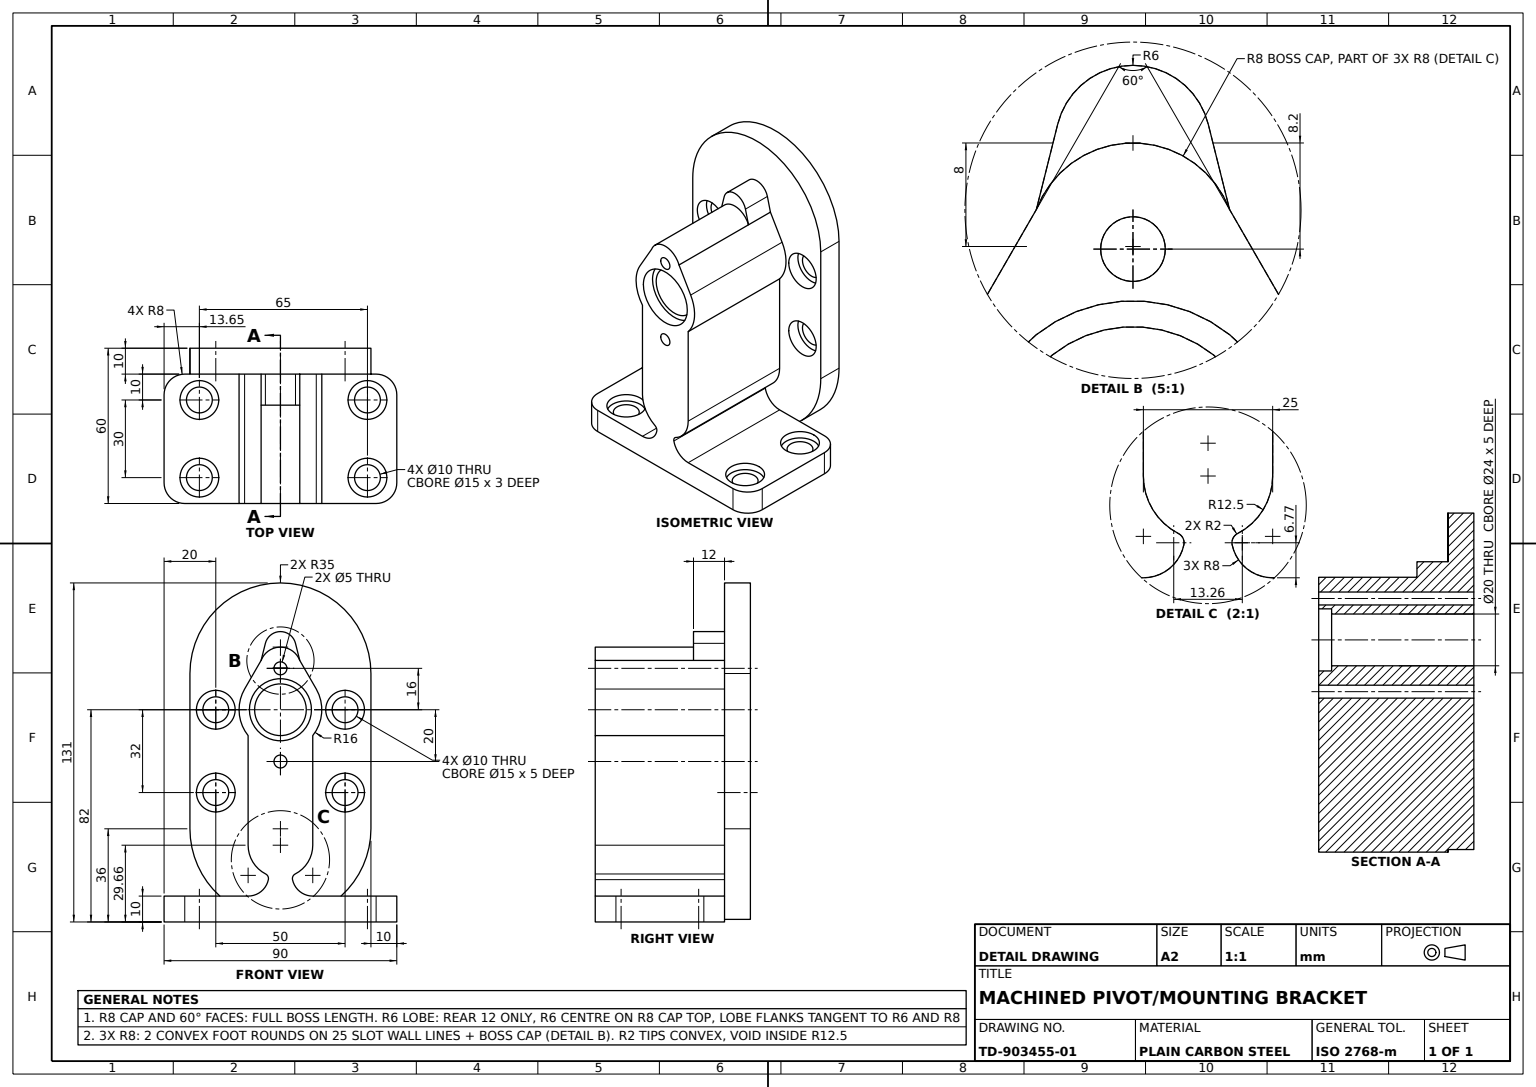
solid
v1 (-16,0,60)
v2 (-16,0,10)
e1 v1 v2 LINE
v3 (-13.856406,8,60)
e2 v3 v1 CIRCLE(AX(P(0,0,60),D(0,0,1),D(1,0,0)),16)
v4 (-13.856406,8,10)
e3 v3 v4 LINE
e4 v4 v2 CIRCLE(AX(P(0,0,10),D(0,0,1),D(1,0,0)),16)
face CYL(AX(P(0,0,60),D(0,0,-1),D(-1,0,0)),16) [-e1 -e2 e3 e4]
v5 (30,0,5)
v6 (20,0,5)
e5 v5 v6 CIRCLE(AX(P(25,0,5),D(0,0,1),D(1,0,0)),5)
e6 v6 v5 CIRCLE(AX(P(25,0,5),D(0,0,1),D(1,0,0)),5)
v7 (32.5,0,5)
v8 (17.5,0,5)
e7 v7 v8 CIRCLE(AX(P(25,0,5),D(0,0,1),D(1,0,0)),7.5)
e8 v8 v7 CIRCLE(AX(P(25,0,5),D(0,0,1),D(1,0,0)),7.5)
face PLANE(AX(P(25,0,5),D(0,0,1),D(1,0,0))) [-e5 -e6] [e7 e8]
v9 (7.473379,19.055728,22)
v10 (7.473379,19.055728,10)
e9 v9 v10 LINE
v11 (5.820364,25.658327,10)
e10 v10 v11 LINE
v12 (5.820364,25.658327,22)
e11 v12 v11 LINE
e12 v9 v12 LINE
face PLANE(AX(P(7.473379,19.055728,22),D(-0.970060689,-0.242862635,0),D(0.242862635,-0.970060689,0))) rev [e9 e10 -e11 -e12]
v13 (2.5,-20,60)
v14 (-2.5,-20,60)
e13 v13 v14 CIRCLE(AX(P(0,-20,60),D(0,0,1),D(1,0,0)),2.5)
e14 v14 v13 CIRCLE(AX(P(0,-20,60),D(0,0,1),D(1,0,0)),2.5)
v15 (-2.5,16,60)
v16 (2.5,16,60)
e15 v15 v16 CIRCLE(AX(P(0,16,60),D(0,0,1),D(1,0,0)),2.5)
e16 v16 v15 CIRCLE(AX(P(0,16,60),D(0,0,1),D(1,0,0)),2.5)
v17 (-12,0,60)
v18 (12,0,60)
e17 v17 v18 CIRCLE(AX(P(0,0,60),D(0,0,1),D(1,0,0)),12)
e18 v18 v17 CIRCLE(AX(P(0,0,60),D(0,0,1),D(1,0,0)),12)
v19 (-37,-72,60)
v20 (-37,-82,60)
e19 v19 v20 LINE
v21 (37,-82,60)
e20 v20 v21 LINE
v22 (37,-72,60)
e21 v21 v22 LINE
v23 (12.5,-72,60)
e22 v22 v23 LINE
v24 (4.671138,-65.645881,60)
e23 v23 v24 CIRCLE(AX(P(12.5,-64,60),D(0,0,-1),D(1,0,0)),8)
v25 (4.628354,-65.234411,60)
e24 v25 v24 CIRCLE(AX(P(6.628354,-65.234411,60),D(0,0,1),D(1,0,0)),2)
v26 (5.714098,-63.455609,60)
e25 v26 v25 CIRCLE(AX(P(6.628354,-65.234411,60),D(0,0,1),D(1,0,0)),2)
v27 (12.5,-52.338096,60)
e26 v27 v26 CIRCLE(AX(P(0,-52.338096,60),D(0,0,-1),D(1,0,0)),12.5)
v28 (12.5,-9.987492,60)
e27 v28 v27 LINE
v29 (13.856406,8,60)
e28 v28 v29 CIRCLE(AX(P(0,0,60),D(0,0,1),D(1,0,0)),16)
v30 (7.473379,19.055728,60)
e29 v30 v29 LINE
v31 (-7.473379,19.055728,60)
e30 v31 v30 CIRCLE(AX(P(0,16.201151,60),D(0,0,-1),D(1,0,0)),8)
e31 v31 v3 LINE
v32 (-12.5,-9.987492,60)
e32 v1 v32 CIRCLE(AX(P(0,0,60),D(0,0,1),D(1,0,0)),16)
v33 (-12.5,-52.338096,60)
e33 v32 v33 LINE
v34 (-5.714098,-63.455609,60)
e34 v33 v34 CIRCLE(AX(P(0,-52.338096,60),D(0,0,1),D(1,0,0)),12.5)
v35 (-4.671138,-65.645881,60)
e35 v34 v35 CIRCLE(AX(P(-6.628354,-65.234411,60),D(0,0,-1),D(1,0,0)),2)
v36 (-12.5,-72,60)
e36 v36 v35 CIRCLE(AX(P(-12.5,-64,60),D(0,0,1),D(1,0,0)),8)
e37 v36 v19 LINE
face PLANE(AX(P(0,0,60),D(0,0,1),D(1,0,0))) [-e13 -e14] [-e15 -e16] [-e17 -e18] [e19 e20 e21 e22 e23 -e24 -e25 -e26 -e27 e28 -e29 -e30 e31 e2 e32 e33 e34 e35 -e36 e37]
v37 (-37,-82,10)
v38 (-37,-72,10)
e38 v37 v38 LINE
v39 (-45,-82,18)
e39 v39 v37 CIRCLE(AX(P(-37,-82,18),D(0,-1,0),D(-1,0,0)),8)
v40 (-45,-72,18)
e40 v40 v39 LINE
e41 v38 v40 CIRCLE(AX(P(-37,-72,18),D(0,1,0),D(0,0,-1)),8)
face CYL(AX(P(-37,0,18),D(0,-1,0),D(1,0,0)),8) [-e38 -e39 -e40 -e41]
v41 (2.5,-20,0)
e42 v13 v41 LINE
v42 (-2.5,-20,0)
e43 v42 v41 CIRCLE(AX(P(0,-20,0),D(0,0,1),D(1,0,0)),2.5)
e44 v14 v42 LINE
face CYL(AX(P(0,-20,60),D(0,0,-1),D(-1,0,0)),2.5) rev [e42 -e43 -e44 e14]
v43 (17.5,-32,5)
v44 (17.5,-32,10)
e45 v43 v44 LINE
v45 (32.5,-32,5)
e46 v45 v43 CIRCLE(AX(P(25,-32,5),D(0,0,1),D(1,0,0)),7.5)
v46 (32.5,-32,10)
e47 v45 v46 LINE
e48 v46 v44 CIRCLE(AX(P(25,-32,10),D(0,0,1),D(1,0,0)),7.5)
face CYL(AX(P(25,-32,5),D(0,0,1),D(1,0,0)),7.5) rev [-e45 -e46 e47 e48]
v47 (-32.5,-32,5)
v48 (-17.5,-32,5)
e49 v47 v48 CIRCLE(AX(P(-25,-32,5),D(0,0,1),D(1,0,0)),7.5)
v49 (-32.5,-32,10)
e50 v47 v49 LINE
v50 (-17.5,-32,10)
e51 v49 v50 CIRCLE(AX(P(-25,-32,10),D(0,0,1),D(1,0,0)),7.5)
e52 v48 v50 LINE
face CYL(AX(P(-25,-32,5),D(0,0,1),D(1,0,0)),7.5) rev [-e49 e50 e51 -e52]
v51 (-17.5,0,10)
v52 (-32.5,0,10)
e53 v51 v52 CIRCLE(AX(P(-25,0,10),D(0,0,1),D(1,0,0)),7.5)
e54 v52 v51 CIRCLE(AX(P(-25,0,10),D(0,0,1),D(1,0,0)),7.5)
v53 (-7.473379,19.055728,10)
e55 v53 v4 LINE
v54 (-5.820364,25.658327,10)
e56 v54 v53 LINE
e57 v11 v54 CIRCLE(AX(P(0,24.201151,10),D(0,0,1),D(1,0,0)),6)
v55 (13.856406,8,10)
e58 v10 v55 LINE
v56 (12.5,-9.987492,10)
e59 v56 v55 CIRCLE(AX(P(0,0,10),D(0,0,1),D(1,0,0)),16)
v57 (12.5,-52.338096,10)
e60 v56 v57 LINE
v58 (5.714098,-63.455609,10)
e61 v57 v58 CIRCLE(AX(P(0,-52.338096,10),D(0,0,-1),D(1,0,0)),12.5)
v59 (4.628354,-65.234411,10)
e62 v58 v59 CIRCLE(AX(P(6.628354,-65.234411,10),D(0,0,1),D(1,0,0)),2)
v60 (4.671138,-65.645881,10)
e63 v59 v60 CIRCLE(AX(P(6.628354,-65.234411,10),D(0,0,1),D(1,0,0)),2)
v61 (12.5,-72,10)
e64 v61 v60 CIRCLE(AX(P(12.5,-64,10),D(0,0,-1),D(1,0,0)),8)
v62 (23.430749,-72,10)
e65 v62 v61 LINE
v63 (35,-46,10)
e66 v62 v63 CIRCLE(AX(P(0,-46,10),D(0,0,1),D(1,0,0)),35)
v64 (35,14,10)
e67 v63 v64 LINE
v65 (-35,14,10)
e68 v64 v65 CIRCLE(AX(P(0,14,10),D(0,0,1),D(-1,0,0)),35)
v66 (-35,-46,10)
e69 v65 v66 LINE
v67 (-23.430749,-72,10)
e70 v66 v67 CIRCLE(AX(P(0,-46,10),D(0,0,1),D(1,0,0)),35)
v68 (-12.5,-72,10)
e71 v68 v67 LINE
v69 (-4.671138,-65.645881,10)
e72 v68 v69 CIRCLE(AX(P(-12.5,-64,10),D(0,0,1),D(1,0,0)),8)
v70 (-5.714098,-63.455609,10)
e73 v70 v69 CIRCLE(AX(P(-6.628354,-65.234411,10),D(0,0,-1),D(1,0,0)),2)
v71 (-12.5,-52.338096,10)
e74 v71 v70 CIRCLE(AX(P(0,-52.338096,10),D(0,0,1),D(1,0,0)),12.5)
v72 (-12.5,-9.987492,10)
e75 v72 v71 LINE
e76 v2 v72 CIRCLE(AX(P(0,0,10),D(0,0,1),D(1,0,0)),16)
e77 v44 v46 CIRCLE(AX(P(25,-32,10),D(0,0,1),D(1,0,0)),7.5)
v73 (32.5,0,10)
v74 (17.5,0,10)
e78 v73 v74 CIRCLE(AX(P(25,0,10),D(0,0,1),D(1,0,0)),7.5)
e79 v74 v73 CIRCLE(AX(P(25,0,10),D(0,0,1),D(1,0,0)),7.5)
e80 v50 v49 CIRCLE(AX(P(-25,-32,10),D(0,0,1),D(1,0,0)),7.5)
face PLANE(AX(P(0,14,10),D(0,0,-1),D(-1,0,0))) rev [-e53 -e54] [-e4 -e55 -e56 -e57 -e10 e58 -e59 e60 e61 e62 e63 -e64 -e65 e66 e67 e68 e69 e70 -e71 e72 -e73 -e74 -e75 -e76] [-e77 -e48] [-e78 -e79] [-e51 -e80]
v75 (45,-72,52)
v76 (45,-72,18)
e81 v75 v76 LINE
v77 (45,-82,52)
e82 v75 v77 LINE
v78 (45,-82,18)
e83 v77 v78 LINE
e84 v78 v76 LINE
face PLANE(AX(P(45,0,60),D(-1,0,0),D(0,-1,0))) rev [-e81 e82 e83 e84]
e85 v25 v59 LINE
e86 v24 v60 LINE
face CYL(AX(P(6.628354,-65.234411,60),D(0,0,-1),D(-1,0,0)),2) rev [-e63 -e85 e24 e86]
v79 (-30,-32,5)
v80 (-20,-32,5)
e87 v79 v80 CIRCLE(AX(P(-25,-32,5),D(0,0,1),D(1,0,0)),5)
e88 v80 v79 CIRCLE(AX(P(-25,-32,5),D(0,0,1),D(1,0,0)),5)
e89 v48 v47 CIRCLE(AX(P(-25,-32,5),D(0,0,1),D(1,0,0)),7.5)
face PLANE(AX(P(-25,-32,5),D(0,0,1),D(1,0,0))) [-e87 -e88] [e89 e49]
v81 (-30,-32,0)
e90 v79 v81 LINE
v82 (-20,-32,0)
e91 v82 v81 CIRCLE(AX(P(-25,-32,0),D(0,0,1),D(1,0,0)),5)
e92 v80 v82 LINE
face CYL(AX(P(-25,-32,10),D(0,0,-1),D(-1,0,0)),5) rev [e90 -e91 -e92 e88]
v83 (37,-82,10)
e93 v83 v78 CIRCLE(AX(P(37,-82,18),D(0,-1,0),D(-1,0,0)),8)
v84 (37,-72,10)
e94 v84 v83 LINE
e95 v76 v84 CIRCLE(AX(P(37,-72,18),D(0,1,0),D(1,0,0)),8)
face CYL(AX(P(37,0,18),D(0,1,0),D(-1,0,0)),8) [-e93 -e94 -e95 -e84]
v85 (-45,-72,52)
e96 v85 v19 CIRCLE(AX(P(-37,-72,52),D(0,1,0),D(0,0,-1)),8)
v86 (-45,-82,52)
e97 v86 v85 LINE
e98 v20 v86 CIRCLE(AX(P(-37,-82,52),D(0,-1,0),D(-1,0,0)),8)
face CYL(AX(P(-37,0,52),D(0,1,0),D(-1,0,0)),8) [-e19 -e96 -e97 -e98]
v87 (-2.5,16,0)
e99 v15 v87 LINE
v88 (2.5,16,0)
e100 v88 v87 CIRCLE(AX(P(0,16,0),D(0,0,1),D(1,0,0)),2.5)
e101 v16 v88 LINE
face CYL(AX(P(0,16,60),D(0,0,-1),D(-1,0,0)),2.5) rev [e16 e99 -e100 -e101]
v89 (-17.5,0,5)
e102 v89 v51 LINE
v90 (-32.5,0,5)
e103 v90 v89 CIRCLE(AX(P(-25,0,5),D(0,0,1),D(1,0,0)),7.5)
e104 v90 v52 LINE
face CYL(AX(P(-25,0,5),D(0,0,1),D(1,0,0)),7.5) rev [-e102 -e103 e104 e54]
v91 (-20,0,0)
v92 (-30,0,0)
e105 v91 v92 CIRCLE(AX(P(-25,0,0),D(0,0,1),D(1,0,0)),5)
v93 (-20,0,5)
e106 v93 v91 LINE
v94 (-30,0,5)
e107 v93 v94 CIRCLE(AX(P(-25,0,5),D(0,0,1),D(1,0,0)),5)
e108 v94 v92 LINE
face CYL(AX(P(-25,0,10),D(0,0,-1),D(-1,0,0)),5) rev [-e105 -e106 e107 e108]
v95 (-7.473379,19.055728,22)
e109 v31 v95 LINE
e110 v95 v53 LINE
face PLANE(AX(P(-13.856406,8,60),D(0.866025404,-0.5,0),D(0.5,0.866025404,0))) rev [e109 e110 e55 -e3 -e31]
v96 (-12,0,55)
e111 v96 v17 LINE
v97 (12,0,55)
e112 v97 v18 LINE
e113 v96 v97 CIRCLE(AX(P(0,0,55),D(0,0,1),D(1,0,0)),12)
face CYL(AX(P(0,0,55),D(0,0,1),D(1,0,0)),12) rev [e111 e17 -e112 -e113]
v98 (33.649744,-75,25)
v99 (33.649744,-75,15)
e114 v98 v99 CIRCLE(AX(P(33.649744,-75,20),D(0,-1,0),D(0,0,1)),5)
v100 (33.649744,-82,25)
e115 v100 v98 LINE
v101 (33.649744,-82,15)
e116 v101 v100 CIRCLE(AX(P(33.649744,-82,20),D(0,1,0),D(-1,0,0)),5)
e117 v101 v99 LINE
face CYL(AX(P(33.649744,-92,20),D(0,1,0),D(0,0,1)),5) rev [-e114 -e115 -e116 e117]
v102 (-35,-46,0)
e118 v66 v102 LINE
v103 (35,-46,0)
e119 v102 v103 CIRCLE(AX(P(0,-46,0),D(0,0,1),D(1,0,0)),35)
e120 v63 v103 LINE
e121 v67 v62 CIRCLE(AX(P(0,-46,10),D(0,0,1),D(1,0,0)),35)
face CYL(AX(P(0,-46,10),D(0,0,-1),D(-1,0,0)),35) [e118 e119 -e120 -e66 -e121 -e70]
face CYL(AX(P(-25,-32,5),D(0,0,1),D(1,0,0)),7.5) rev [e52 e80 -e50 -e89]
v104 (30,0,0)
e122 v5 v104 LINE
v105 (20,0,0)
e123 v105 v104 CIRCLE(AX(P(25,0,0),D(0,0,1),D(1,0,0)),5)
e124 v6 v105 LINE
face CYL(AX(P(25,0,10),D(0,0,-1),D(-1,0,0)),5) rev [e6 e122 -e123 -e124]
v106 (-31.350256,-75,12.5)
v107 (-31.350256,-75,27.5)
e125 v106 v107 CIRCLE(AX(P(-31.350256,-75,20),D(0,1,0),D(0,0,1)),7.5)
v108 (-31.350256,-72,12.5)
e126 v106 v108 LINE
v109 (-31.350256,-72,27.5)
e127 v108 v109 CIRCLE(AX(P(-31.350256,-72,20),D(0,1,0),D(0,0,1)),7.5)
e128 v107 v109 LINE
face CYL(AX(P(-31.350256,-75,20),D(0,1,0),D(0,0,1)),7.5) rev [-e125 e126 e127 -e128]
v110 (-5.820364,25.658327,22)
e129 v110 v95 LINE
e130 v95 v9 CIRCLE(AX(P(0,16.201151,22),D(0,0,-1),D(-1,0,0)),8)
e131 v12 v110 CIRCLE(AX(P(0,24.201151,22),D(0,0,1),D(1,0,0)),6)
face PLANE(AX(P(0,16.201151,22),D(0,0,-1),D(-1,0,0))) rev [e129 e130 e12 e131]
e132 v100 v101 CIRCLE(AX(P(33.649744,-82,20),D(0,1,0),D(-1,0,0)),5)
e133 v99 v98 CIRCLE(AX(P(33.649744,-75,20),D(0,-1,0),D(0,0,1)),5)
face CYL(AX(P(33.649744,-92,20),D(0,1,0),D(0,0,1)),5) rev [-e117 -e132 e115 -e133]
v111 (33.649744,-75,12.5)
v112 (33.649744,-75,27.5)
e134 v111 v112 CIRCLE(AX(P(33.649744,-75,20),D(0,1,0),D(0,0,1)),7.5)
e135 v112 v111 CIRCLE(AX(P(33.649744,-75,20),D(0,1,0),D(0,0,1)),7.5)
face PLANE(AX(P(33.649744,-75,20),D(0,1,0),D(0,0,1))) [e134 e135] [e133 e114]
v113 (-31.350256,-75,57.5)
v114 (-31.350256,-75,42.5)
e136 v113 v114 CIRCLE(AX(P(-31.350256,-75,50),D(0,1,0),D(0,0,1)),7.5)
v115 (-31.350256,-72,57.5)
e137 v113 v115 LINE
v116 (-31.350256,-72,42.5)
e138 v115 v116 CIRCLE(AX(P(-31.350256,-72,50),D(0,1,0),D(0,0,1)),7.5)
e139 v114 v116 LINE
face CYL(AX(P(-31.350256,-75,50),D(0,1,0),D(0,0,1)),7.5) rev [-e136 e137 e138 -e139]
e140 v27 v57 LINE
e141 v26 v58 LINE
face CYL(AX(P(0,-52.338096,60),D(0,0,-1),D(-1,0,0)),12.5) [-e61 -e140 e26 e141]
v117 (35,14,0)
e142 v64 v117 LINE
e143 v103 v117 LINE
face PLANE(AX(P(35,-46,10),D(-1,0,0),D(0,-1,0))) rev [-e142 -e67 e120 e143]
e144 v30 v9 LINE
face CYL(AX(P(0,16.201151,60),D(0,0,-1),D(-1,0,0)),8) [-e130 -e109 e30 e144]
e145 v89 v90 CIRCLE(AX(P(-25,0,5),D(0,0,1),D(1,0,0)),7.5)
face CYL(AX(P(-25,0,5),D(0,0,1),D(1,0,0)),7.5) rev [-e104 -e145 e102 e53]
e146 v114 v113 CIRCLE(AX(P(-31.350256,-75,50),D(0,1,0),D(0,0,1)),7.5)
v118 (-31.350256,-75,45)
v119 (-31.350256,-75,55)
e147 v118 v119 CIRCLE(AX(P(-31.350256,-75,50),D(0,-1,0),D(0,0,1)),5)
e148 v119 v118 CIRCLE(AX(P(-31.350256,-75,50),D(0,-1,0),D(0,0,1)),5)
face PLANE(AX(P(-31.350256,-75,50),D(0,1,0),D(0,0,1))) [e146 e136] [e147 e148]
v120 (30,-32,5)
v121 (30,-32,0)
e149 v120 v121 LINE
v122 (20,-32,5)
e150 v120 v122 CIRCLE(AX(P(25,-32,5),D(0,0,1),D(1,0,0)),5)
v123 (20,-32,0)
e151 v122 v123 LINE
e152 v121 v123 CIRCLE(AX(P(25,-32,0),D(0,0,1),D(1,0,0)),5)
face CYL(AX(P(25,-32,10),D(0,0,-1),D(-1,0,0)),5) rev [-e149 e150 e151 -e152]
e153 v81 v82 CIRCLE(AX(P(-25,-32,0),D(0,0,1),D(1,0,0)),5)
face CYL(AX(P(-25,-32,10),D(0,0,-1),D(-1,0,0)),5) rev [-e153 -e90 e87 e92]
e154 v92 v91 CIRCLE(AX(P(-25,0,0),D(0,0,1),D(1,0,0)),5)
e155 v94 v93 CIRCLE(AX(P(-25,0,5),D(0,0,1),D(1,0,0)),5)
face CYL(AX(P(-25,0,10),D(0,0,-1),D(-1,0,0)),5) rev [e106 -e154 -e108 e155]
e156 v35 v69 LINE
e157 v36 v68 LINE
face CYL(AX(P(-12.5,-64,60),D(0,0,-1),D(-1,0,0)),8) rev [e36 e156 -e72 -e157]
e158 v97 v96 CIRCLE(AX(P(0,0,55),D(0,0,1),D(1,0,0)),12)
face CYL(AX(P(0,0,55),D(0,0,1),D(1,0,0)),12) rev [-e111 -e158 e112 e18]
e159 v33 v71 LINE
e160 v34 v70 LINE
face CYL(AX(P(0,-52.338096,60),D(0,0,-1),D(-1,0,0)),12.5) [-e34 e159 e74 -e160]
e161 v109 v108 CIRCLE(AX(P(-31.350256,-72,20),D(0,1,0),D(0,0,1)),7.5)
e162 v107 v106 CIRCLE(AX(P(-31.350256,-75,20),D(0,1,0),D(0,0,1)),7.5)
face CYL(AX(P(-31.350256,-75,20),D(0,1,0),D(0,0,1)),7.5) rev [e161 -e126 -e162 e128]
v124 (33.649744,-82,45)
v125 (33.649744,-82,55)
e163 v124 v125 CIRCLE(AX(P(33.649744,-82,50),D(0,1,0),D(-1,0,0)),5)
v126 (33.649744,-75,45)
e164 v124 v126 LINE
v127 (33.649744,-75,55)
e165 v127 v126 CIRCLE(AX(P(33.649744,-75,50),D(0,-1,0),D(0,0,1)),5)
e166 v125 v127 LINE
face CYL(AX(P(33.649744,-92,50),D(0,1,0),D(0,0,1)),5) rev [-e163 e164 -e165 -e166]
e167 v104 v105 CIRCLE(AX(P(25,0,0),D(0,0,1),D(1,0,0)),5)
face CYL(AX(P(25,0,10),D(0,0,-1),D(-1,0,0)),5) rev [-e167 -e122 e5 e124]
v128 (10,0,55)
v129 (-10,0,55)
e168 v128 v129 CIRCLE(AX(P(0,0,55),D(0,0,1),D(1,0,0)),10)
e169 v129 v128 CIRCLE(AX(P(0,0,55),D(0,0,1),D(1,0,0)),10)
face PLANE(AX(P(0,0,55),D(0,0,1),D(1,0,0))) [e158 e113] [-e168 -e169]
e170 v126 v127 CIRCLE(AX(P(33.649744,-75,50),D(0,-1,0),D(0,0,1)),5)
e171 v125 v124 CIRCLE(AX(P(33.649744,-82,50),D(0,1,0),D(-1,0,0)),5)
face CYL(AX(P(33.649744,-92,50),D(0,1,0),D(0,0,1)),5) rev [e166 -e170 -e164 -e171]
e172 v23 v61 LINE
face CYL(AX(P(12.5,-64,60),D(0,0,-1),D(-1,0,0)),8) rev [-e86 -e23 e172 e64]
e173 v28 v56 LINE
face PLANE(AX(P(12.5,0,60),D(1,0,0),D(0,1,0))) [-e60 -e173 e27 e140]
face PLANE(AX(P(-25,0,5),D(0,0,1),D(1,0,0))) [e103 e145] [-e155 -e107]
e174 v7 v73 LINE
e175 v8 v74 LINE
face CYL(AX(P(25,0,5),D(0,0,1),D(1,0,0)),7.5) rev [e174 e78 -e175 -e7]
v130 (-31.350256,-82,25)
v131 (-31.350256,-75,25)
e176 v130 v131 LINE
v132 (-31.350256,-82,15)
e177 v132 v130 CIRCLE(AX(P(-31.350256,-82,20),D(0,1,0),D(-1,0,0)),5)
v133 (-31.350256,-75,15)
e178 v132 v133 LINE
e179 v131 v133 CIRCLE(AX(P(-31.350256,-75,20),D(0,-1,0),D(0,0,1)),5)
face CYL(AX(P(-31.350256,-92,20),D(0,1,0),D(0,0,1)),5) rev [-e176 -e177 e178 -e179]
e180 v110 v54 LINE
face CYL(AX(P(0,24.201151,22),D(0,0,-1),D(-1,0,0)),6) [-e131 e11 e57 -e180]
v134 (-31.350256,-82,55)
e181 v134 v119 LINE
v135 (-31.350256,-82,45)
e182 v135 v118 LINE
e183 v134 v135 CIRCLE(AX(P(-31.350256,-82,50),D(0,1,0),D(-1,0,0)),5)
face CYL(AX(P(-31.350256,-92,50),D(0,1,0),D(0,0,1)),5) rev [e181 -e147 -e182 -e183]
e184 v29 v55 LINE
face CYL(AX(P(0,0,60),D(0,0,-1),D(-1,0,0)),16) [-e28 e173 e59 -e184]
v136 (-35,14,0)
e185 v65 v136 LINE
e186 v136 v102 LINE
face PLANE(AX(P(-35,-46,10),D(1,0,0),D(0,1,0))) rev [e185 e186 -e118 -e69]
v137 (33.649744,-75,57.5)
v138 (33.649744,-75,42.5)
e187 v137 v138 CIRCLE(AX(P(33.649744,-75,50),D(0,1,0),D(0,0,1)),7.5)
e188 v138 v137 CIRCLE(AX(P(33.649744,-75,50),D(0,1,0),D(0,0,1)),7.5)
face PLANE(AX(P(33.649744,-75,50),D(0,1,0),D(0,0,1))) [e170 e165] [e187 e188]
e189 v32 v72 LINE
face CYL(AX(P(0,0,60),D(0,0,-1),D(-1,0,0)),16) [-e32 e1 e76 -e189]
face CYL(AX(P(6.628354,-65.234411,60),D(0,0,-1),D(-1,0,0)),2) rev [-e141 e25 e85 -e62]
face PLANE(AX(P(-12.5,0,60),D(1,0,0),D(0,1,0))) rev [-e159 -e33 e189 e75]
v139 (33.649744,-72,42.5)
v140 (33.649744,-72,57.5)
e190 v139 v140 CIRCLE(AX(P(33.649744,-72,50),D(0,1,0),D(0,0,1)),7.5)
e191 v137 v140 LINE
e192 v138 v139 LINE
face CYL(AX(P(33.649744,-75,50),D(0,1,0),D(0,0,1)),7.5) rev [e190 -e191 -e188 e192]
e193 v67 v38 LINE
e194 v84 v62 LINE
e195 v37 v83 LINE
face PLANE(AX(P(0,0,10),D(0,0,1),D(1,0,0))) rev [-e193 e121 -e194 e94 -e195 e38]
e196 v117 v136 CIRCLE(AX(P(0,14,0),D(0,0,1),D(-1,0,0)),35)
face CYL(AX(P(0,14,10),D(0,0,-1),D(-1,0,0)),35) [-e185 -e68 e142 e196]
e197 v133 v131 CIRCLE(AX(P(-31.350256,-75,20),D(0,-1,0),D(0,0,1)),5)
face PLANE(AX(P(-31.350256,-75,20),D(0,1,0),D(0,0,1))) [e162 e125] [e197 e179]
e198 v43 v45 CIRCLE(AX(P(25,-32,5),D(0,0,1),D(1,0,0)),7.5)
face CYL(AX(P(25,-32,5),D(0,0,1),D(1,0,0)),7.5) rev [e77 -e47 -e198 e45]
face CYL(AX(P(25,0,5),D(0,0,1),D(1,0,0)),7.5) rev [-e8 e175 e79 -e174]
e199 v86 v39 LINE
e200 v85 v40 LINE
face PLANE(AX(P(-45,0,60),D(1,0,0),D(0,1,0))) rev [-e199 e97 e200 e40]
e201 v77 v21 CIRCLE(AX(P(37,-82,52),D(0,-1,0),D(-1,0,0)),8)
e202 v135 v134 CIRCLE(AX(P(-31.350256,-82,50),D(0,1,0),D(-1,0,0)),5)
e203 v130 v132 CIRCLE(AX(P(-31.350256,-82,20),D(0,1,0),D(-1,0,0)),5)
face PLANE(AX(P(0,-82,60),D(0,1,0),D(-1,0,0))) rev [e163 e171] [e132 e116] [e93 -e83 e201 -e20 e98 e199 e39 e195] [e202 e183] [e177 e203]
face CYL(AX(P(-6.628354,-65.234411,60),D(0,0,-1),D(-1,0,0)),2) rev [e73 -e156 -e35 e160]
v141 (33.649744,-72,12.5)
e204 v111 v141 LINE
v142 (33.649744,-72,27.5)
e205 v141 v142 CIRCLE(AX(P(33.649744,-72,20),D(0,1,0),D(0,0,1)),7.5)
e206 v112 v142 LINE
face CYL(AX(P(33.649744,-75,20),D(0,1,0),D(0,0,1)),7.5) rev [e204 e205 -e206 -e134]
e207 v142 v141 CIRCLE(AX(P(33.649744,-72,20),D(0,1,0),D(0,0,1)),7.5)
face CYL(AX(P(33.649744,-75,20),D(0,1,0),D(0,0,1)),7.5) rev [e206 e207 -e204 -e135]
e208 v41 v42 CIRCLE(AX(P(0,-20,0),D(0,0,1),D(1,0,0)),2.5)
face CYL(AX(P(0,-20,60),D(0,0,-1),D(-1,0,0)),2.5) rev [-e208 -e42 e13 e44]
e209 v116 v115 CIRCLE(AX(P(-31.350256,-72,50),D(0,1,0),D(0,0,1)),7.5)
face CYL(AX(P(-31.350256,-75,50),D(0,1,0),D(0,0,1)),7.5) rev [-e146 e139 e209 -e137]
v143 (10,0,0)
e210 v128 v143 LINE
v144 (-10,0,0)
e211 v143 v144 CIRCLE(AX(P(0,0,0),D(0,0,-1),D(-1,0,0)),10)
e212 v129 v144 LINE
face CYL(AX(P(0,0,60),D(0,0,-1),D(-1,0,0)),10) rev [e210 e211 -e212 e169]
e213 v122 v120 CIRCLE(AX(P(25,-32,5),D(0,0,1),D(1,0,0)),5)
e214 v123 v121 CIRCLE(AX(P(25,-32,0),D(0,0,1),D(1,0,0)),5)
face CYL(AX(P(25,-32,10),D(0,0,-1),D(-1,0,0)),5) rev [-e151 e213 e149 -e214]
face CYL(AX(P(-31.350256,-92,20),D(0,1,0),D(0,0,1)),5) rev [e176 -e197 -e178 -e203]
e215 v144 v143 CIRCLE(AX(P(0,0,0),D(0,0,-1),D(-1,0,0)),10)
face CYL(AX(P(0,0,60),D(0,0,-1),D(-1,0,0)),10) rev [e212 e215 -e210 e168]
e216 v140 v139 CIRCLE(AX(P(33.649744,-72,50),D(0,1,0),D(0,0,1)),7.5)
e217 v22 v75 CIRCLE(AX(P(37,-72,52),D(0,1,0),D(1,0,0)),8)
face PLANE(AX(P(0,-72,60),D(0,-1,0),D(1,0,0))) rev [-e207 -e205] [-e216 -e190] [e95 e194 e65 -e172 -e22 e217 e81]
face PLANE(AX(P(0,-72,60),D(0,-1,0),D(0,0,-1))) rev [-e161 -e127] [-e138 -e209] [e193 e41 -e200 e96 -e37 e157 e71]
face CYL(AX(P(-31.350256,-92,50),D(0,1,0),D(0,0,1)),5) rev [-e181 -e202 e182 -e148]
face CYL(AX(P(33.649744,-75,50),D(0,1,0),D(0,0,1)),7.5) rev [e191 e216 -e192 -e187]
e218 v87 v88 CIRCLE(AX(P(0,16,0),D(0,0,1),D(1,0,0)),2.5)
face CYL(AX(P(0,16,60),D(0,0,-1),D(-1,0,0)),2.5) rev [e101 -e218 -e99 e15]
face CYL(AX(P(37,0,52),D(0,-1,0),D(1,0,0)),8) [-e21 -e201 -e82 -e217]
face PLANE(AX(P(13.856406,8,60),D(0.866025404,0.5,0),D(-0.5,0.866025404,0))) [-e9 -e144 e29 e184 -e58]
face PLANE(AX(P(0,14,0),D(0,0,-1),D(-1,0,0))) [e105 e154] [e214 e152] [-e215 -e211] [-e186 -e196 -e143 -e119] [e208 e43] [e91 e153] [e100 e218] [e167 e123]
face PLANE(AX(P(25,-32,5),D(0,0,1),D(1,0,0))) [-e150 -e213] [e46 e198]
face PLANE(AX(P(-7.473379,19.055728,22),D(0.970060689,-0.242862635,0),D(0.242862635,0.970060689,0))) rev [e180 e56 -e110 -e129]
